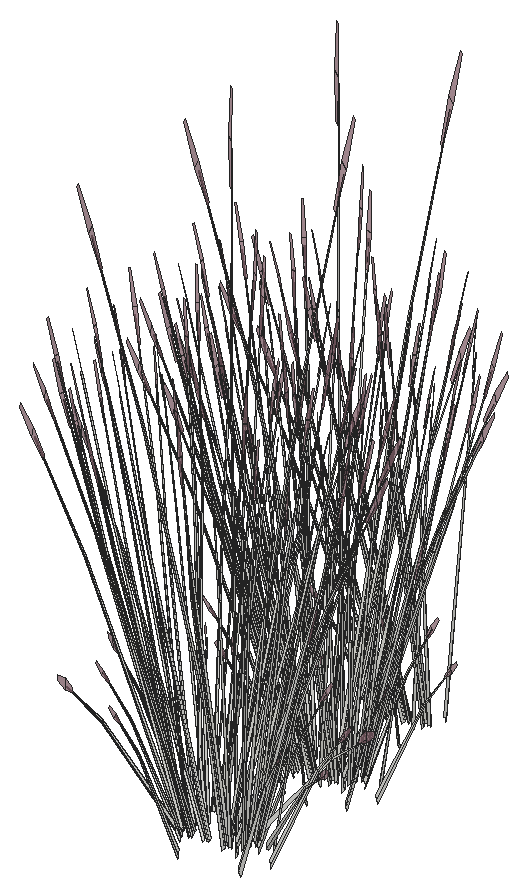
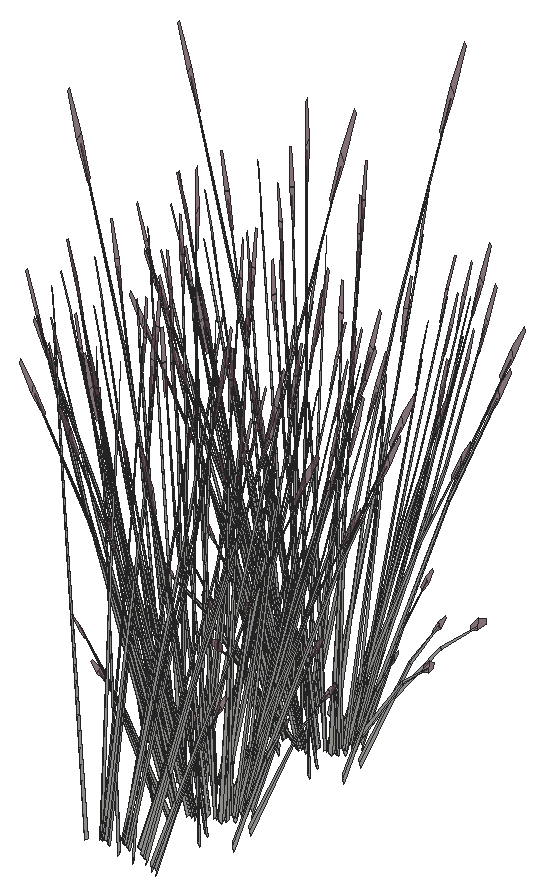
# SketchUp Ruby script. Lengths in inches.
U = 1.inch
M = Sketchup.active_model
def pt(a) = Geom::Point3d.new(a.map { |v| v * U })
def face(e, loops, mat)
  f = e.add_face(loops[0].map { |a| pt(a) })
  loops[1..].each { |l| e.add_face(l.map { |a| pt(a) }).erase! }
  f.material = f.back_material = mat if mat
  f
end
# faces: each face lists its corners as indices into pts; further lists are holes
def faces(e, pts, list, mat = nil) = list.each { |f| face(e, (f[0].is_a?(Array) ? f : [f]).map { |l| l.map { |i| pts[i] } }, mat) }
# xy, xz, yz: faces in a plane at the given z, y or x. An outline is a flat list of corners, or four numbers for a rectangle; further outlines are holes
def ring(l) = l.size == 4 ? [[l[0], l[1]], [l[2], l[1]], [l[2], l[3]], [l[0], l[3]]] : l.each_slice(2).to_a
def flat(e, list, mat, &to3) = list.each { |f| face(e, (f[0].is_a?(Array) ? f : [f]).map { |l| ring(l).map { |u, v| to3.(u, v) } }, mat) }
def xy(e, z, list, mat = nil) = flat(e, list, mat) { |x, y| [x, y, z] }
def xz(e, y, list, mat = nil) = flat(e, list, mat) { |x, z| [x, y, z] }
def yz(e, x, list, mat = nil) = flat(e, list, mat) { |y, z| [x, y, z] }
def lines(e, pts, list) = list.each { |a, b| e.add_line(pt(pts[a]), pt(pts[b])) }
# prism: a flat outline (further loops are holes) pulled along v
def prism(e, loops, v, mat = nil)
  f = face(e, loops, mat); d = Geom::Vector3d.new(v.map { |x| x * U })
  f.pushpull(f.normal.samedirection?(d) ? d.length : -d.length)
end
def box(e, o, s, mat = nil) = prism(e, [[o, [o[0] + s[0], o[1], o[2]], [o[0] + s[0], o[1] + s[1], o[2]], [o[0], o[1] + s[1], o[2]]]], [0, 0, s[2]], mat)
def at(x, y, z, deg = 0) = Geom::Transformation.translation(pt([x, y, z])) * Geom::Transformation.rotation(ORIGIN, Z_AXIS, deg.degrees)
def axes(o, x, y, z) = Geom::Transformation.new([*x, 0, *y, 0, *z, 0, *pt(o).to_a, 1])
def part(name) = M.definitions.add(name)
# library, detail: a bought-in or finely detailed component or shape, given as its bounding box
def library(name, o, s) = part(name).tap { |d| box(d.entities, o, s) }
def detail(e, o, s) = box(e.add_group.entities, o, s)
def put(e, d, t, mat = nil) = e.add_instance(d, t).tap { |i| i.material = mat if mat }
def group(e, t, mat = nil) = e.add_group.tap { |g| g.transformation = t; g.material = mat if mat }.entities
root = M.entities
M.materials.add("LightPink_Translucent").color = [144, 107, 117]
M.materials["LightPink_Translucent"].alpha = 0.75
c1 = part("blade")
p = [[2.15,0.21,22],[0,0.17,0],[0.09,0.45,0],[2.18,0.31,22],[2.29,0.31,22],[0.38,0.45,0],
  [2.48,0.24,33],[2.49,0.24,33],[2.48,0.22,33]]
faces(c1.entities,p,[[0,1,2,3],[4,5,2,3],[6,3,4,7],[8,0,3,6]])
c2 = part("seeds")
p = [[0.3,-0.1,1.38],[-0.01,-0.03,1.59],[-0.01,-0.03,0.03],[0.14,-0.07,-0.07],[0.29,-0.03,3],[0.15,0.01,3.11]]
faces(c2.entities,p,[[0,1,2,3],[1,0,4,5]],"LightPink_Translucent")
c3 = part("blade with seeds")
put(c3.entities,c1,at(0,0,0))
put(c3.entities,c2,axes([2.4,0.25,30.99],[1.5799,-0.05474,1.17369],[-0.12525,1.92788,0.29478],[-0.07173,-0.02425,1.56792]))
put(root,c3,axes([335.01,385.74,52.14],[-0.36145,-0.26255,-0.45151],[0.38183,-0.22994,-0.34973],[0.055,-0.1334,0.86392]))
put(root,c3,axes([334.36,385.47,52.45],[-0.49409,0.18193,-0.10745],[-0.24281,-0.32289,-0.59638],[-0.06519,-0.13607,0.90619]))
put(root,c3,axes([335.38,385.88,52.45],[-0.55492,-0.01936,-0.10745],[0.01517,-0.36657,-0.59638],[0.03855,-0.14118,0.90619]))
put(root,c3,axes([335.35,385.64,52],[0.34164,-0.20573,-0.31292],[0.3234,0.23491,0.40398],[0.04921,-0.11936,0.77298]))
put(root,c3,axes([332.39,384.92,50.44],[0.26338,0.136,1.01491],[-0.38358,0.08175,0.74569],[-0.08207,-0.10452,0.22354]))
put(root,c3,axes([333.03,385.64,52.4],[-0.43054,-0.18887,-0.62776],[0.30598,-0.33097,0.07576],[-0.15599,-0.11277,0.88802]))
put(root,c3,axes([332.88,385.39,52],[-0.07798,-0.31474,-0.31292],[0.44579,-0.08311,0.40398],[-0.11974,-0.09019,0.77298]))
put(root,c3,axes([331.92,385.85,51.43],[0.18755,0.06732,1.51428],[-0.38813,0.28243,0.12244],[-0.24191,-0.12741,0.64734]))
put(root,c3,axes([332.83,385.65,52.14],[-0.49824,0.09289,-0.45151],[-0.08716,-0.35177,-0.34973],[-0.13382,-0.10081,0.86392]))
put(root,c3,axes([335.77,386.49,52.4],[0.26374,-0.30832,-0.62776],[0.46217,0.21911,0.07576],[0.15748,-0.11171,0.88802]))
put(root,c3,axes([335.76,386.34,52.14],[-0.12971,-0.3568,-0.45151],[0.49122,-0.06241,-0.34973],[0.14077,-0.09583,0.86392]))
put(root,c3,axes([331.88,385.23,52.17],[-0.10864,-0.00276,1.54581],[-0.34587,0.27582,-0.24447],[-0.18454,-0.05636,0.12397]))
put(root,c3,axes([335.99,386.6,52.45],[-0.46706,-0.21546,-0.10745],[0.26908,-0.31203,-0.59638],[0.13196,-0.10846,0.90619]))
put(root,c3,axes([334.06,387.78,50.9375],[0.43633,0.15757,1.33654],[-0.42745,0.33945,0.52853],[-0.19146,-0.20119,1.12046]))
put(root,c3,axes([336.36,385.63,50.44],[-0.16818,0.19891,1.01491],[-0.14456,-0.26725,0.74569],[0.1389,-0.06697,0.22354]))
put(root,c3,axes([336.12,386.38,52],[0.43951,-0.05584,-0.31292],[0.11606,0.31924,0.40398],[0.12595,-0.08575,0.77298]))
put(root,c3,axes([331.85,385.94,52],[-0.28729,-0.24465,-0.31292],[0.32804,-0.23159,0.40398],[-0.16667,-0.03524,0.77298]))
put(root,c3,axes([332.15,386.11,52.4],[-0.50473,-0.00941,-0.62776],[0.0339,-0.39618,0.07576],[-0.21383,-0.04181,0.88802]))
put(root,c3,axes([337.39,386.89,52.17],[0.07006,-0.05952,1.54581],[-0.08968,-0.3651,-0.24447],[0.1758,-0.06922,0.12397]))
put(root,c3,axes([331.98,386.1875,52.14],[-0.36663,0.25884,-0.45151],[-0.32109,-0.27343,-0.34973],[-0.18628,-0.03938,0.86392]))
put(root,c3,axes([331.16,386.53,50.44],[0.32236,-0.02796,1.01491],[-0.20448,0.24636,0.74569],[-0.1593,-0.03696,0.22354]))
put(root,c3,axes([332.18,385.92,52.45],[-0.02704,0.39739,-0.10745],[-0.51189,-0.01086,-0.59638],[-0.19715,-0.0276,0.90619]))
put(root,c3,axes([336.01,387.44,52.45],[-0.25405,-0.35383,-0.10745],[0.45089,-0.17388,-0.59638],[0.19001,-0.04668,0.90619]))
put(root,c3,axes([335.98,387.14,52.14],[0.13679,-0.35544,-0.45151],[0.46898,0.12183,-0.34973],[0.18882,-0.03259,0.86392]))
put(root,c3,axes([331.52,386.46,51.43],[0.20943,-0.00885,1.51428],[-0.13893,0.38357,0.12244],[-0.29846,-0.02372,0.64734]))
put(root,c3,axes([335.9,387.27,52.4],[0.44368,-0.17257,-0.62776],[0.24726,0.35524,0.07576],[0.21437,-0.04035,0.88802]))
put(root,c3,axes([336.27,387.3,52],[0.41962,0.10901,-0.31292],[-0.12239,0.31802,0.40398],[0.16894,-0.02916,0.77298]))
put(root,c3,axes([331.34,386.79,52],[-0.41962,-0.10901,-0.31292],[0.12239,-0.31802,0.40398],[-0.16894,0.02916,0.77298]))
put(root,c3,axes([335.13,386.91,51.43],[-0.20943,0.00885,1.51428],[0.13893,-0.38357,0.12244],[0.29846,0.02372,0.64734]))
put(root,c3,axes([332.62,386.74,50.95],[0.14352,-0.05653,1.56454],[0.04949,0.39467,0.12244],[-0.31087,0.05237,0.55918]))
put(root,c3,axes([337.16,387.36,50.44],[-0.31197,0.06451,1.01491],[0.14684,-0.26661,0.74569],[0.1655,0.01824,0.22354]))
put(root,c3,axes([331.08,387,52.17],[-0.08245,0.05073,1.54581],[0.00701,0.37067,-0.24447],[-0.18899,0.0482,0.12397]))
put(root,c3,axes([331.63,386.95,52.14],[-0.13679,0.35544,-0.45151],[-0.46898,-0.12183,-0.34973],[-0.18882,0.03259,0.86392]))
put(root,c3,axes([331.61,386.65,52.45],[0.25405,0.35383,-0.10745],[-0.45089,0.17388,-0.59638],[-0.19001,0.04668,0.90619]))
put(root,c3,axes([336.62,388.1875,51.47],[-0.09664,-0.32847,-0.03085],[0.45676,-0.07551,-0.13989],[0.09538,0.02082,0.4614]))
put(root,c3,axes([335.4375,388.18,52.45],[0.02704,-0.39739,-0.10745],[0.51189,0.01086,-0.59638],[0.19715,0.0276,0.90619]))
put(root,c3,axes([335.88,387.9375,52.17],[0.10831,-0.00661,1.54581],[0.29709,-0.30358,-0.24447],[0.19266,0.04007,0.12397]))
put(root,c3,axes([331.61,387.14,51.43],[0.17519,-0.08265,1.51428],[0.14749,0.38193,0.12244],[-0.27504,0.08632,0.64734]))
put(root,c3,axes([335.46,387.98,52.4],[0.50473,0.00941,-0.62776],[-0.0339,0.39618,0.07576],[0.21383,0.04181,0.88802]))
put(root,c3,axes([330.7,388.48,50.44],[0.21042,-0.1771,1.01491],[0.08303,0.28036,0.74569],[-0.15207,0.0502,0.22354]))
put(root,c3,axes([335.77,388.15,52],[0.28729,0.24465,-0.31292],[-0.32804,0.23159,0.40398],[0.16667,0.03524,0.77298]))
put(root,c3,axes([331.49,387.71,52],[-0.43951,0.05584,-0.31292],[-0.11606,-0.31924,0.40398],[-0.12595,0.08575,0.77298]))
put(root,c3,axes([334.73,387.52,51.43],[-0.18755,-0.06732,1.51428],[0.38813,-0.28243,0.12244],[0.24191,0.12741,0.64734]))
put(root,c3,axes([334.77,386.63,51.95],[-0.4363,-0.20303,1.22187],[0.46069,-0.31611,0.5272],[0.14077,0.1905,1.18105]))
put(root,c3,axes([331.625,387.49,52.45],[0.46706,0.21546,-0.10745],[-0.26908,0.31203,-0.59638],[-0.13196,0.10846,0.90619]))
put(root,c3,axes([335.43,388.29,50.44],[-0.28429,-0.11236,1.01491],[0.36709,-0.11416,0.74569],[0.09901,0.0967,0.22354]))
put(root,c3,axes([334.43,388.61,52.45],[0.30087,-0.33447,-0.10745],[0.43572,0.19269,-0.59638],[0.15146,0.0945,0.90619]))
put(root,c3,axes([332.25,387.4,51.43],[0.12611,-0.12006,1.51428],[0.31843,0.32408,0.12244],[-0.2184,0.14759,0.64734]))
put(root,c3,axes([331.86,387.75,52.14],[0.12971,0.3568,-0.45151],[-0.49122,0.06241,-0.34973],[-0.14077,0.09583,0.86392]))
put(root,c3,axes([334.74,387.02,50.51],[-0.01379,-0.36791,1.24828],[0.62424,0.09537,0.52853],[-0.14764,0.20132,1.17828]))
put(root,c3,axes([334.79,388.44,52.14],[0.49824,-0.09289,-0.45151],[0.08716,0.35177,-0.34973],[0.13382,0.10081,0.86392]))
put(root,c3,axes([332.16,387.69,51.43],[0.09401,-0.13431,1.51428],[0.3944,0.27795,0.12244],[-0.17792,0.17323,0.64734]))
put(root,c3,axes([332.27,388.45,52],[-0.34164,0.20573,-0.31292],[-0.3234,-0.23491,0.40398],[-0.04921,0.11936,0.77298]))
put(root,c3,axes([331.09,388.39,52.17],[-0.01255,0.07733,1.54581],[0.35618,0.269,-0.24447],[-0.09325,0.12721,0.12397]))
put(root,c3,axes([333.25,388.62,52.45],[0.49409,-0.18193,-0.10745],[0.24281,0.32289,-0.59638],[0.06519,0.13607,0.90619]))
put(root,c3,axes([332.48,389.25,50.44],[-0.01307,-0.23234,1.01491],[0.32652,0.16572,0.74569],[-0.06422,0.11074,0.22354]))
put(root,c3,axes([332.61,388.35,52.42],[0.36145,0.26255,-0.50118],[-0.38183,0.22994,-0.3882],[-0.055,0.1334,0.95895]))
put(root,c3,axes([333.68,388.61,52.14],[0.49634,0.09796,-0.45151],[-0.17013,0.33585,-0.34973],[0.04551,0.13522,0.86392]))
put(root,c3,axes([333.96,387.91,51.43],[-0.11542,-0.12546,1.51428],[0.53333,-0.10562,0.12244],[0.12054,0.19696,0.64734]))
put(root,c3,axes([333.45,388.8125,52],[-0.15222,0.30049,-0.31292],[-0.44409,-0.08764,0.40398],[0.04072,0.12098,0.77298]))
put(root,c3,axes([332.49,388.23,52.72],[-0.01314,0.36145,-0.69681],[-0.55324,-0.02428,0.08409],[-0.05838,0.15313,0.9857]))
put(root,c3,axes([333.02,387.97,51.43],[-0.01236,-0.14998,1.51428],[0.53562,0.09949,0.12244],[-0.03313,0.21373,0.64734]))
put(root,c3,axes([332.69,395.14,51.43],[0.11542,0.12546,1.51428],[-0.53333,0.10562,0.12244],[-0.12054,-0.19696,0.64734]))
put(root,c3,axes([333.5,388.54,52.4],[0.24099,0.31773,-0.62776],[-0.49607,0.17707,0.07576],[0.05635,0.15352,0.88802]))
put(root,c3,axes([333.14,389.34,52.17],[0.064,0.06292,1.54581],[0.51651,0.02472,-0.24447],[0.05194,0.13877,0.12397]))
put(root,c3,axes([334.11,395.23,52.4],[-0.24099,-0.31773,-0.62776],[0.49607,-0.17707,0.07576],[-0.05635,-0.15352,0.88802]))
put(root,c3,axes([335.12,395.54,52.4],[0.01314,-0.36145,-0.62776],[0.55324,0.02428,0.07576],[0.05838,-0.15313,0.88802]))
put(root,c3,axes([334.16,394.96,52],[0.15222,-0.30049,-0.31292],[0.44409,0.08764,0.40398],[-0.04072,-0.12098,0.77298]))
put(root,c3,axes([334.5,395.36,51.43],[-0.09401,0.13431,1.51428],[-0.3944,-0.27795,0.12244],[0.17792,-0.17323,0.64734]))
put(root,c3,axes([332.31,388.74,50.97],[0.01109,-0.20172,1.3638],[0.49896,0.10655,0.18846],[-0.04323,0.21498,0.64398]))
put(root,c3,axes([333.93,395.17,52.14],[-0.49634,-0.09796,-0.45151],[0.17013,-0.33585,-0.34973],[-0.04551,-0.13522,0.86392]))
put(root,c3,axes([334.24,394.33,50.44],[0.06477,0.22786,1.01491],[-0.35932,-0.1262,0.74569],[0.03867,-0.11667,0.22354]))
put(root,c3,axes([335.01,395.42,52.14],[-0.36145,-0.26255,-0.45151],[0.38183,-0.22994,-0.34973],[0.055,-0.1334,0.86392]))
put(root,c3,axes([334.36,395.15,52.45],[-0.49409,0.18193,-0.10745],[-0.24281,-0.32289,-0.59638],[-0.06519,-0.13607,0.90619]))
put(root,c3,axes([335.38,395.56,52.45],[-0.55492,-0.01936,-0.10745],[0.01517,-0.36657,-0.59638],[0.03855,-0.14118,0.90619]))
put(root,c3,axes([335.35,395.32,52],[0.34164,-0.20573,-0.31292],[0.3234,0.23491,0.40398],[0.04921,-0.11936,0.77298]))
put(root,c3,axes([332.39,394.6,50.44],[0.26338,0.136,1.01491],[-0.38358,0.08175,0.74569],[-0.08207,-0.10452,0.22354]))
put(root,c3,axes([333.03,395.32,52.4],[-0.43054,-0.18887,-0.62776],[0.30598,-0.33097,0.07576],[-0.15599,-0.11277,0.88802]))
put(root,c3,axes([332.88,395.07,52],[-0.07798,-0.31474,-0.31292],[0.44579,-0.08311,0.40398],[-0.11974,-0.09019,0.77298]))
put(root,c3,axes([331.92,395.53,51.43],[0.18755,0.06732,1.51428],[-0.38813,0.28243,0.12244],[-0.24191,-0.12741,0.64734]))
put(root,c3,axes([332.83,395.33,52.14],[-0.49824,0.09289,-0.45151],[-0.08716,-0.35177,-0.34973],[-0.13382,-0.10081,0.86392]))
put(root,c3,axes([335.77,396.17,52.4],[0.26374,-0.30832,-0.62776],[0.46217,0.21911,0.07576],[0.15748,-0.11171,0.88802]))
put(root,c3,axes([335.76,396.03,52.14],[-0.12971,-0.3568,-0.45151],[0.49122,-0.06241,-0.34973],[0.14077,-0.09583,0.86392]))
put(root,c3,axes([335.99,396.28,52.45],[-0.46706,-0.21546,-0.10745],[0.26908,-0.31203,-0.59638],[0.13196,-0.10846,0.90619]))
put(root,c3,axes([334.06,397.46,50.9375],[0.43633,0.15757,1.33654],[-0.42745,0.33945,0.52853],[-0.19146,-0.20119,1.12046]))
put(root,c3,axes([336.36,395.32,50.44],[-0.16818,0.19891,1.01491],[-0.14456,-0.26725,0.74569],[0.1389,-0.06697,0.22354]))
put(root,c3,axes([336.12,396.0625,52],[0.43951,-0.05584,-0.31292],[0.11606,0.31924,0.40398],[0.12595,-0.08575,0.77298]))
put(root,c3,axes([331.85,395.625,52],[-0.28729,-0.24465,-0.31292],[0.32804,-0.23159,0.40398],[-0.16667,-0.03524,0.77298]))
put(root,c3,axes([332.15,395.79,52.4],[-0.50473,-0.00941,-0.62776],[0.0339,-0.39618,0.07576],[-0.21383,-0.04181,0.88802]))
put(root,c3,axes([331.98,395.87,52.14],[-0.36663,0.25884,-0.45151],[-0.32109,-0.27343,-0.34973],[-0.18628,-0.03938,0.86392]))
put(root,c3,axes([331.16,396.21,50.44],[0.32236,-0.02796,1.01491],[-0.20448,0.24636,0.74569],[-0.1593,-0.03696,0.22354]))
put(root,c3,axes([332.18,395.6,52.45],[-0.02704,0.39739,-0.10745],[-0.51189,-0.01086,-0.59638],[-0.19715,-0.0276,0.90619]))
put(root,c3,axes([336.01,397.12,52.45],[-0.25405,-0.35383,-0.10745],[0.45089,-0.17388,-0.59638],[0.19001,-0.04668,0.90619]))
put(root,c3,axes([335.98,396.82,52.14],[0.13679,-0.35544,-0.45151],[0.46898,0.12183,-0.34973],[0.18882,-0.03259,0.86392]))
put(root,c3,axes([331.52,396.14,51.43],[0.20943,-0.00885,1.51428],[-0.13893,0.38357,0.12244],[-0.29846,-0.02372,0.64734]))
put(root,c3,axes([335.9,396.95,52.4],[0.44368,-0.17257,-0.62776],[0.24726,0.35524,0.07576],[0.21437,-0.04035,0.88802]))
put(root,c3,axes([336.27,396.98,52],[0.41962,0.10901,-0.31292],[-0.12239,0.31802,0.40398],[0.16894,-0.02916,0.77298]))
put(root,c3,axes([331.34,396.47,52],[-0.41962,-0.10901,-0.31292],[0.12239,-0.31802,0.40398],[-0.16894,0.02916,0.77298]))
put(root,c3,axes([335.13,396.59,51.43],[-0.20943,0.00885,1.51428],[0.13893,-0.38357,0.12244],[0.29846,0.02372,0.64734]))
put(root,c3,axes([332.62,396.42,50.95],[0.14352,-0.05653,1.56454],[0.04949,0.39467,0.12244],[-0.31087,0.05237,0.55918]))
put(root,c3,axes([337.16,397.04,50.44],[-0.31197,0.06451,1.01491],[0.14684,-0.26661,0.74569],[0.1655,0.01824,0.22354]))
put(root,c3,axes([331.63,396.64,52.14],[-0.13679,0.35544,-0.45151],[-0.46898,-0.12183,-0.34973],[-0.18882,0.03259,0.86392]))
put(root,c3,axes([331.61,396.33,52.45],[0.25405,0.35383,-0.10745],[-0.45089,0.17388,-0.59638],[-0.19001,0.04668,0.90619]))
put(root,c3,axes([336.62,397.87,51.47],[-0.09664,-0.32847,-0.03085],[0.45676,-0.07551,-0.13989],[0.09538,0.02082,0.4614]))
put(root,c3,axes([335.4375,397.86,52.45],[0.02704,-0.39739,-0.10745],[0.51189,0.01086,-0.59638],[0.19715,0.0276,0.90619]))
put(root,c3,axes([331.61,396.82,51.43],[0.17519,-0.08265,1.51428],[0.14749,0.38193,0.12244],[-0.27504,0.08632,0.64734]))
put(root,c3,axes([335.46,397.67,52.4],[0.50473,0.00941,-0.62776],[-0.0339,0.39618,0.07576],[0.21383,0.04181,0.88802]))
put(root,c3,axes([330.7,398.16,50.44],[0.21042,-0.1771,1.01491],[0.08303,0.28036,0.74569],[-0.15207,0.0502,0.22354]))
put(root,c3,axes([335.77,397.83,52],[0.28729,0.24465,-0.31292],[-0.32804,0.23159,0.40398],[0.16667,0.03524,0.77298]))
put(root,c3,axes([331.49,397.39,52],[-0.43951,0.05584,-0.31292],[-0.11606,-0.31924,0.40398],[-0.12595,0.08575,0.77298]))
put(root,c3,axes([334.73,397.2,51.43],[-0.18755,-0.06732,1.51428],[0.38813,-0.28243,0.12244],[0.24191,0.12741,0.64734]))
put(root,c3,axes([334.77,396.32,51.95],[-0.4363,-0.20303,1.22187],[0.46069,-0.31611,0.5272],[0.14077,0.1905,1.18105]))
put(root,c3,axes([331.625,397.17,52.45],[0.46706,0.21546,-0.10745],[-0.26908,0.31203,-0.59638],[-0.13196,0.10846,0.90619]))
put(root,c3,axes([335.43,397.97,50.44],[-0.28429,-0.11236,1.01491],[0.36709,-0.11416,0.74569],[0.09901,0.0967,0.22354]))
put(root,c3,axes([334.43,398.29,52.45],[0.30087,-0.33447,-0.10745],[0.43572,0.19269,-0.59638],[0.15146,0.0945,0.90619]))
put(root,c3,axes([332.25,397.08,51.43],[0.12611,-0.12006,1.51428],[0.31843,0.32408,0.12244],[-0.2184,0.14759,0.64734]))
put(root,c3,axes([331.86,397.43,52.14],[0.12971,0.3568,-0.45151],[-0.49122,0.06241,-0.34973],[-0.14077,0.09583,0.86392]))
put(root,c3,axes([334.74,396.7,50.51],[-0.01379,-0.36791,1.24828],[0.62424,0.09537,0.52853],[-0.14764,0.20132,1.17828]))
put(root,c3,axes([334.79,398.125,52.14],[0.49824,-0.09289,-0.45151],[0.08716,0.35177,-0.34973],[0.13382,0.10081,0.86392]))
put(root,c3,axes([332.69,403.6,51.43],[0.11542,0.12546,1.51428],[-0.53333,0.10562,0.12244],[-0.12054,-0.19696,0.64734]))
put(root,c3,axes([332.16,397.37,51.43],[0.09401,-0.13431,1.51428],[0.3944,0.27795,0.12244],[-0.17792,0.17323,0.64734]))
put(root,c3,axes([334.11,403.69,52.4],[-0.24099,-0.31773,-0.62776],[0.49607,-0.17707,0.07576],[-0.05635,-0.15352,0.88802]))
put(root,c3,axes([332.27,398.13,52],[-0.34164,0.20573,-0.31292],[-0.3234,-0.23491,0.40398],[-0.04921,0.11936,0.77298]))
put(root,c3,axes([333.25,398.3,52.45],[0.49409,-0.18193,-0.10745],[0.24281,0.32289,-0.59638],[0.06519,0.13607,0.90619]))
put(root,c3,axes([332.48,398.93,50.44],[-0.01307,-0.23234,1.01491],[0.32652,0.16572,0.74569],[-0.06422,0.11074,0.22354]))
put(root,c3,axes([335.12,404,52.4],[0.01314,-0.36145,-0.62776],[0.55324,0.02428,0.07576],[0.05838,-0.15313,0.88802]))
put(root,c3,axes([334.16,403.42,52],[0.15222,-0.30049,-0.31292],[0.44409,0.08764,0.40398],[-0.04072,-0.12098,0.77298]))
put(root,c3,axes([334.5,403.82,51.43],[-0.09401,0.13431,1.51428],[-0.3944,-0.27795,0.12244],[0.17792,-0.17323,0.64734]))
put(root,c3,axes([332.61,398.03,52.42],[0.36145,0.26255,-0.50118],[-0.38183,0.22994,-0.3882],[-0.055,0.1334,0.95895]))
put(root,c3,axes([333.68,398.29,52.14],[0.49634,0.09796,-0.45151],[-0.17013,0.33585,-0.34973],[0.04551,0.13522,0.86392]))
put(root,c3,axes([333.96,397.59,51.43],[-0.11542,-0.12546,1.51428],[0.53333,-0.10562,0.12244],[0.12054,0.19696,0.64734]))
put(root,c3,axes([333.93,403.63,52.14],[-0.49634,-0.09796,-0.45151],[0.17013,-0.33585,-0.34973],[-0.04551,-0.13522,0.86392]))
put(root,c3,axes([334.24,402.79,50.44],[0.06477,0.22786,1.01491],[-0.35932,-0.1262,0.74569],[0.03867,-0.11667,0.22354]))
put(root,c3,axes([335.01,403.88,52.14],[-0.36145,-0.26255,-0.45151],[0.38183,-0.22994,-0.34973],[0.055,-0.1334,0.86392]))
put(root,c3,axes([333.45,398.49,52],[-0.15222,0.30049,-0.31292],[-0.44409,-0.08764,0.40398],[0.04072,0.12098,0.77298]))
put(root,c3,axes([332.49,397.91,52.72],[-0.01314,0.36145,-0.69681],[-0.55324,-0.02428,0.08409],[-0.05838,0.15313,0.9857]))
put(root,c3,axes([333.02,397.66,51.43],[-0.01236,-0.14998,1.51428],[0.53562,0.09949,0.12244],[-0.03313,0.21373,0.64734]))
put(root,c3,axes([334.36,403.61,52.45],[-0.49409,0.18193,-0.10745],[-0.24281,-0.32289,-0.59638],[-0.06519,-0.13607,0.90619]))
put(root,c3,axes([335.38,404.02,52.45],[-0.55492,-0.01936,-0.10745],[0.01517,-0.36657,-0.59638],[0.03855,-0.14118,0.90619]))
put(root,c3,axes([335.35,403.79,52],[0.34164,-0.20573,-0.31292],[0.3234,0.23491,0.40398],[0.04921,-0.11936,0.77298]))
put(root,c3,axes([332.39,403.0625,50.44],[0.26338,0.136,1.01491],[-0.38358,0.08175,0.74569],[-0.08207,-0.10452,0.22354]))
put(root,c3,axes([333.03,403.78,52.4],[-0.43054,-0.18887,-0.62776],[0.30598,-0.33097,0.07576],[-0.15599,-0.11277,0.88802]))
put(root,c3,axes([332.88,403.53,52],[-0.07798,-0.31474,-0.31292],[0.44579,-0.08311,0.40398],[-0.11974,-0.09019,0.77298]))
put(root,c3,axes([333.5,398.22,52.4],[0.24099,0.31773,-0.62776],[-0.49607,0.17707,0.07576],[0.05635,0.15352,0.88802]))
put(root,c3,axes([331.92,403.99,51.43],[0.18755,0.06732,1.51428],[-0.38813,0.28243,0.12244],[-0.24191,-0.12741,0.64734]))
put(root,c3,axes([332.83,403.79,52.14],[-0.49824,0.09289,-0.45151],[-0.08716,-0.35177,-0.34973],[-0.13382,-0.10081,0.86392]))
put(root,c3,axes([332.31,398.42,50.97],[0.01109,-0.20172,1.3638],[0.49896,0.10655,0.18846],[-0.04323,0.21498,0.64398]))
put(root,c3,axes([335.77,404.63,52.4],[0.26374,-0.30832,-0.62776],[0.46217,0.21911,0.07576],[0.15748,-0.11171,0.88802]))
